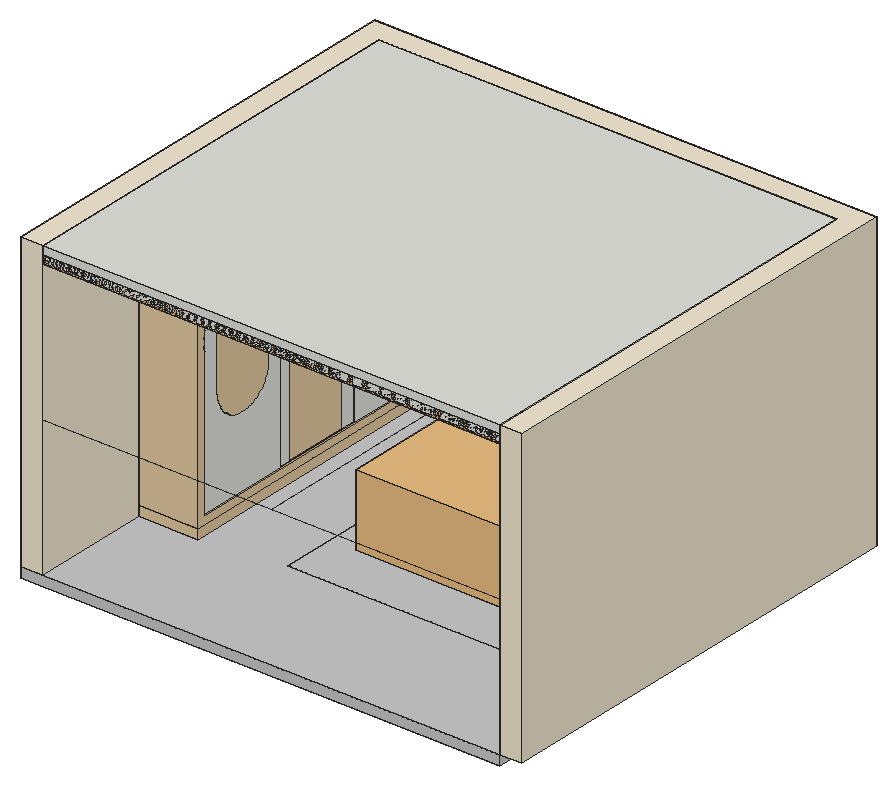
# SketchUp Ruby script. Lengths in inches.
U = 1.inch
M = Sketchup.active_model
def pt(a) = Geom::Point3d.new(a.map { |v| v * U })
def face(e, loops, mat)
  f = e.add_face(loops[0].map { |a| pt(a) })
  loops[1..].each { |l| e.add_face(l.map { |a| pt(a) }).erase! }
  f.material = f.back_material = mat if mat
  f
end
# faces: each face lists its corners as indices into pts; further lists are holes
def faces(e, pts, list, mat = nil) = list.each { |f| face(e, (f[0].is_a?(Array) ? f : [f]).map { |l| l.map { |i| pts[i] } }, mat) }
# xy, xz, yz: faces in a plane at the given z, y or x. An outline is a flat list of corners, or four numbers for a rectangle; further outlines are holes
def ring(l) = l.size == 4 ? [[l[0], l[1]], [l[2], l[1]], [l[2], l[3]], [l[0], l[3]]] : l.each_slice(2).to_a
def flat(e, list, mat, &to3) = list.each { |f| face(e, (f[0].is_a?(Array) ? f : [f]).map { |l| ring(l).map { |u, v| to3.(u, v) } }, mat) }
def xy(e, z, list, mat = nil) = flat(e, list, mat) { |x, y| [x, y, z] }
def xz(e, y, list, mat = nil) = flat(e, list, mat) { |x, z| [x, y, z] }
def yz(e, x, list, mat = nil) = flat(e, list, mat) { |y, z| [x, y, z] }
def lines(e, pts, list) = list.each { |a, b| e.add_line(pt(pts[a]), pt(pts[b])) }
# prism: a flat outline (further loops are holes) pulled along v
def prism(e, loops, v, mat = nil)
  f = face(e, loops, mat); d = Geom::Vector3d.new(v.map { |x| x * U })
  f.pushpull(f.normal.samedirection?(d) ? d.length : -d.length)
end
def box(e, o, s, mat = nil) = prism(e, [[o, [o[0] + s[0], o[1], o[2]], [o[0] + s[0], o[1] + s[1], o[2]], [o[0], o[1] + s[1], o[2]]]], [0, 0, s[2]], mat)
def at(x, y, z, deg = 0) = Geom::Transformation.translation(pt([x, y, z])) * Geom::Transformation.rotation(ORIGIN, Z_AXIS, deg.degrees)
def axes(o, x, y, z) = Geom::Transformation.new([*x, 0, *y, 0, *z, 0, *pt(o).to_a, 1])
def part(name) = M.definitions.add(name)
# library, detail: a bought-in or finely detailed component or shape, given as its bounding box
def library(name, o, s) = part(name).tap { |d| box(d.entities, o, s) }
def detail(e, o, s) = box(e.add_group.entities, o, s)
def put(e, d, t, mat = nil) = e.add_instance(d, t).tap { |i| i.material = mat if mat }
def group(e, t, mat = nil) = e.add_group.tap { |g| g.transformation = t; g.material = mat if mat }.entities
root = M.entities
M.materials.add("0961 AP 7892 PALE IVORY").color = [243, 232, 209]
M.materials.add("0962 AP 9878 Bamboo Straw-N").color = [228, 203, 161]
M.materials.add("Acquerello Marble (TJ07TT)").color = [202, 201, 200]
M.materials.add("Emissive").color = [255, 238, 203]
M.materials.add("Generic").color = [255, 255, 255]
M.materials.add("Kit Kat Speckle_ Stack (OYOLJ5)").color = [227, 224, 217]
M.materials.add("The Belden Brick Company Dapple Gray Matt None Modular (3-5-").color = [200, 200, 200]
M.materials.add("[0130_Gainsboro]").color = [220, 220, 220]
c1 = library("Bed 001",[-37.84,-46.07,0],[75.19,90.39,37.01])
c2 = library("Side Table",[0,-0.77,-1.18],[23.62,18.49,23.93])
c3 = part("Group105\#1")
p = [[0,0,0],[0,0,-46.23],[-14.28,0,-46.23],[93,-56.66,0],[-93,-56.66,0],[93,56.66,0],
  [93,0,0],[-93,56.66,0],[14.28,0,-46.23],[-93,0,0],[0,0,-74.83]]
lines(c3.entities,p,[[0,1],[1,2],[3,4],[5,6],[7,5],[1,8],[9,0],[0,6],[8,10],[4,9],[6,3],[2,10],
  [9,7]])
c4 = part("Rectangle Light\#1")
put(c4.entities,c3,at(0,0,0))
c5 = library("Spot Light",[-5.1,-5.1,-11.05],[10.2,10.2,11.05])
c6 = part("plafonjera+p5")
g1 = group(c6.entities,at(102.27,51.27,12.6))
xy(g1,0,[[[1.84,0,1.6,0.03,1.36,0.09,1.13,0.18,0.91,0.3,0.71,0.45,0.53,0.62,0.375,0.81,0.24,1.02,0.14,1.24,0.0625,1.48,0.02,1.72,0,1.96,0.02,2.21,0.0625,2.45,0.14,2.6875,0.24,2.91,0.375,3.12,0.53,3.3125,0.71,3.48,0.91,3.625,1.13,3.75,1.36,3.84,1.6,3.9,1.84,3.93,2.09,3.93,2.34,3.9,2.58,3.84,2.81,3.75,3.02,3.625,3.22,3.48,3.4,3.3125,3.5625,3.12,3.69,2.91,3.8,2.6875,3.875,2.45,3.92,2.21,3.9375,1.96,3.92,1.72,3.875,1.48,3.8,1.24,3.69,1.02,3.5625,0.81,3.4,0.62,3.22,0.45,3.02,0.3,2.81,0.18,2.58,0.09,2.34,0.03,2.09,0],[1.86,0.2,2.08,0.2,2.3,0.22,2.52,0.28,2.72,0.36,2.92,0.47,3.1,0.6,3.26,0.75,3.4,0.92,3.52,1.11,3.62,1.3125,3.68,1.52,3.73,1.74,3.74,1.96,3.73,2.1875,3.68,2.41,3.62,2.62,3.52,2.82,3.4,3.01,3.26,3.18,3.1,3.33,2.92,3.46,2.72,3.57,2.52,3.65,2.3,3.7,2.08,3.73,1.86,3.73,1.64,3.7,1.42,3.65,1.21,3.57,1.02,3.46,0.84,3.33,0.68,3.18,0.54,3.01,0.42,2.82,0.32,2.62,0.25,2.41,0.21,2.1875,0.2,1.96,0.21,1.74,0.25,1.52,0.32,1.3125,0.42,1.11,0.54,0.92,0.68,0.75,0.84,0.6,1.02,0.47,1.21,0.36,1.42,0.28,1.64,0.22]]],"[0130_Gainsboro]")
xy(g1,0.08,[[1.86,0.2,1.64,0.22,1.42,0.28,1.21,0.36,1.02,0.47,0.84,0.6,0.68,0.75,0.54,0.92,0.42,1.11,0.32,1.3125,0.25,1.52,0.21,1.74,0.2,1.96,0.21,2.1875,0.25,2.41,0.32,2.62,0.42,2.82,0.54,3.01,0.68,3.18,0.84,3.33,1.02,3.46,1.21,3.57,1.42,3.65,1.64,3.7,1.86,3.73,2.08,3.73,2.3,3.7,2.52,3.65,2.72,3.57,2.92,3.46,3.1,3.33,3.26,3.18,3.4,3.01,3.52,2.82,3.62,2.62,3.68,2.41,3.73,2.1875,3.74,1.96,3.73,1.74,3.68,1.52,3.62,1.3125,3.52,1.11,3.4,0.92,3.26,0.75,3.1,0.6,2.92,0.47,2.72,0.36,2.52,0.28,2.3,0.22,2.08,0.2]],"Emissive")
xy(g1,0.39,[[1.84,0,2.09,0,2.34,0.03,2.58,0.09,2.81,0.18,3.02,0.3,3.22,0.45,3.4,0.62,3.5625,0.81,3.69,1.02,3.8,1.24,3.875,1.48,3.92,1.72,3.9375,1.96,3.92,2.21,3.875,2.45,3.8,2.6875,3.69,2.91,3.5625,3.12,3.4,3.3125,3.22,3.48,3.02,3.625,2.81,3.75,2.58,3.84,2.34,3.9,2.09,3.93,1.84,3.93,1.6,3.9,1.36,3.84,1.13,3.75,0.91,3.625,0.71,3.48,0.53,3.3125,0.375,3.12,0.24,2.91,0.14,2.6875,0.0625,2.45,0.02,2.21,0,1.96,0.02,1.72,0.0625,1.48,0.14,1.24,0.24,1.02,0.375,0.81,0.53,0.62,0.71,0.45,0.91,0.3,1.13,0.18,1.36,0.09,1.6,0.03]],"[0130_Gainsboro]")
xz(g1,0,[[1.84,0,2.09,0.39]],"[0130_Gainsboro]")
xz(g1,0.2,[[1.86,0,2.08,0.08]],"[0130_Gainsboro]")
xz(g1,3.73,[[1.86,0,2.08,0.08]],"[0130_Gainsboro]")
xz(g1,3.93,[[1.84,0,2.09,0.39]],"[0130_Gainsboro]")
p = [[1.36,0.09,0],[1.6,0.03,0],[1.6,0.03,0.39],[1.36,0.09,0.39],[1.84,0,0],[1.84,0,0.39],
  [2.09,0,0],[2.34,0.03,0],[2.34,0.03,0.39],[2.09,0,0.39],[2.58,0.09,0],[2.58,0.09,0.39],
  [1.13,0.18,0],[1.13,0.18,0.39],[2.81,0.18,0],[2.81,0.18,0.39],[0.91,0.3,0],[0.91,0.3,0.39],
  [1.64,0.22,0],[1.42,0.28,0],[1.42,0.28,0.08],[1.64,0.22,0.08],[1.86,0.2,0],[1.86,0.2,0.08],
  [2.3,0.22,0],[2.08,0.2,0],[2.08,0.2,0.08],[2.3,0.22,0.08],[2.52,0.28,0],[2.52,0.28,0.08],
  [3.02,0.3,0],[3.02,0.3,0.39],[0.71,0.45,0],[0.71,0.45,0.39],[1.21,0.36,0],[1.21,0.36,0.08],
  [2.72,0.36,0],[2.72,0.36,0.08],[3.22,0.45,0],[3.22,0.45,0.39],[0.53,0.62,0],[0.53,0.62,0.39],
  [1.02,0.47,0],[1.02,0.47,0.08],[2.92,0.47,0],[2.92,0.47,0.08],[3.4,0.62,0],[3.4,0.62,0.39],
  [0.84,0.6,0],[0.84,0.6,0.08],[3.1,0.6,0],[3.1,0.6,0.08],[0.375,0.81,0],[0.375,0.81,0.39],
  [0.68,0.75,0],[0.68,0.75,0.08],[3.26,0.75,0],[3.26,0.75,0.08],[3.5625,0.81,0],[3.5625,0.81,0.39],
  [0.24,1.02,0],[0.24,1.02,0.39],[0.54,0.92,0],[0.54,0.92,0.08],[3.4,0.92,0],[3.4,0.92,0.08],
  [3.69,1.02,0],[3.69,1.02,0.39],[0.42,1.11,0],[0.42,1.11,0.08],[3.52,1.11,0],[3.52,1.11,0.08],
  [0.14,1.24,0],[0.14,1.24,0.39],[3.8,1.24,0],[3.8,1.24,0.39],[0.32,1.3125,0],[0.32,1.3125,0.08],
  [3.62,1.3125,0],[3.62,1.3125,0.08],[0.0625,1.48,0],[0.0625,1.48,0.39],[3.875,1.48,0],[3.875,1.48,0.39],
  [0.25,1.52,0],[0.25,1.52,0.08],[3.68,1.52,0],[3.68,1.52,0.08],[0.02,1.72,0],[0.02,1.72,0.39],
  [0.21,1.74,0],[0.21,1.74,0.08],[3.73,1.74,0],[3.73,1.74,0.08],[3.92,1.72,0],[3.92,1.72,0.39],
  [0,1.96,0],[0,1.96,0.39],[0.2,1.96,0],[0.2,1.96,0.08],[3.74,1.96,0],[3.74,1.96,0.08],
  [3.9375,1.96,0],[3.9375,1.96,0.39],[0.02,2.21,0],[0.02,2.21,0.39],[0.21,2.1875,0],[0.21,2.1875,0.08],
  [3.73,2.1875,0],[3.73,2.1875,0.08],[3.92,2.21,0],[3.92,2.21,0.39],[0.0625,2.45,0],[0.0625,2.45,0.39],
  [0.25,2.41,0],[0.25,2.41,0.08],[3.68,2.41,0],[3.68,2.41,0.08],[3.875,2.45,0],[3.875,2.45,0.39],
  [0.32,2.62,0],[0.32,2.62,0.08],[3.62,2.62,0],[3.62,2.62,0.08],[0.14,2.6875,0],[0.14,2.6875,0.39],
  [3.8,2.6875,0],[3.8,2.6875,0.39],[0.42,2.82,0],[0.42,2.82,0.08],[3.52,2.82,0],[3.52,2.82,0.08],
  [0.24,2.91,0],[0.24,2.91,0.39],[3.69,2.91,0],[3.69,2.91,0.39],[0.54,3.01,0],[0.54,3.01,0.08],
  [3.4,3.01,0],[3.4,3.01,0.08],[0.375,3.12,0],[0.375,3.12,0.39],[3.5625,3.12,0],[3.5625,3.12,0.39],
  [0.68,3.18,0],[0.68,3.18,0.08],[3.26,3.18,0],[3.26,3.18,0.08],[0.53,3.3125,0],[0.53,3.3125,0.39],
  [3.4,3.3125,0],[3.4,3.3125,0.39],[0.84,3.33,0],[0.84,3.33,0.08],[3.1,3.33,0],[3.1,3.33,0.08],
  [0.71,3.48,0],[0.71,3.48,0.39],[1.02,3.46,0],[1.02,3.46,0.08],[2.92,3.46,0],[2.92,3.46,0.08],
  [3.22,3.48,0],[3.22,3.48,0.39],[0.91,3.625,0],[0.91,3.625,0.39],[1.21,3.57,0],[1.21,3.57,0.08],
  [2.72,3.57,0],[2.72,3.57,0.08],[3.02,3.625,0],[3.02,3.625,0.39],[1.13,3.75,0],[1.13,3.75,0.39],
  [1.42,3.65,0],[1.42,3.65,0.08],[1.64,3.7,0],[1.64,3.7,0.08],[2.3,3.7,0],[2.52,3.65,0],
  [2.52,3.65,0.08],[2.3,3.7,0.08],[2.81,3.75,0],[2.81,3.75,0.39],[1.36,3.84,0],[1.36,3.84,0.39],
  [1.86,3.73,0],[1.86,3.73,0.08],[2.08,3.73,0],[2.08,3.73,0.08],[2.58,3.84,0],[2.58,3.84,0.39],
  [1.6,3.9,0],[1.6,3.9,0.39],[2.34,3.9,0],[2.34,3.9,0.39],[1.84,3.93,0],[1.84,3.93,0.39],
  [2.09,3.93,0],[2.09,3.93,0.39]]
faces(g1,p,[[0,1,2,3],[1,4,5,2],[6,7,8,9],[7,10,11,8],[12,0,3,13],[10,14,15,11],[16,12,13,17],[18,19,20,21],
  [22,18,21,23],[24,25,26,27],[28,24,27,29],[14,30,31,15],[32,16,17,33],[19,34,35,20],[36,28,29,37],[30,38,39,31],
  [40,32,33,41],[34,42,43,35],[44,36,37,45],[38,46,47,39],[42,48,49,43],[50,44,45,51],[52,40,41,53],[48,54,55,49],
  [56,50,51,57],[46,58,59,47],[60,52,53,61],[54,62,63,55],[64,56,57,65],[58,66,67,59],[62,68,69,63],[70,64,65,71],
  [72,60,61,73],[66,74,75,67],[68,76,77,69],[78,70,71,79],[80,72,73,81],[74,82,83,75],[76,84,85,77],[86,78,79,87],
  [88,80,81,89],[84,90,91,85],[92,86,87,93],[82,94,95,83],[96,88,89,97],[90,98,99,91],[100,92,93,101],[94,102,103,95],
  [104,96,97,105],[98,106,107,99],[108,100,101,109],[102,110,111,103],[112,104,105,113],[106,114,115,107],[116,108,109,117],[110,118,119,111],
  [114,120,121,115],[122,116,117,123],[124,112,113,125],[118,126,127,119],[120,128,129,121],[130,122,123,131],[132,124,125,133],[126,134,135,127],
  [128,136,137,129],[138,130,131,139],[140,132,133,141],[134,142,143,135],[136,144,145,137],[146,138,139,147],[148,140,141,149],[142,150,151,143],
  [144,152,153,145],[154,146,147,155],[156,148,149,157],[152,158,159,153],[160,154,155,161],[150,162,163,151],[164,156,157,165],[158,166,167,159],
  [168,160,161,169],[162,170,171,163],[172,164,165,173],[166,174,175,167],[174,176,177,175],[178,179,180,181],[179,168,169,180],[170,182,183,171],
  [184,172,173,185],[176,186,187,177],[188,178,181,189],[182,190,191,183],[192,184,185,193],[190,194,195,191],[196,192,193,197],[194,198,199,195]],"[0130_Gainsboro]")
put(g1,c5,at(1.89,2.02,0.07))
c7 = library("ceiling fan",[0,0,0],[76.25,93.13,30.02])
c8 = part("fan")
p = [[217.53,-902.72,540.32],[217.53,-902.72,540.32],[217.53,-902.72,541.35],[217.53,-902.72,541.35]]
lines(c8.entities,p,[[0,1],[2,3]])
put(c8.entities,c7,at(256.45,-350.9,679.41))
c9 = library("Group\#4",[-0.5,-1.92,0],[127,2.42,36])
c10 = library("Group\#18",[-0.5,-0.5,0],[151,1.71,48])
c11 = part("Group8\#1")
xy(c11.entities,7,[[-26.93,80.42,-2.93,81.13],[-26.93,109.26,-2.93,109.97],[-26.93,138.1,-2.93,138.81]])
xy(c11.entities,42.65,[[-26.93,51.9375,-2.93,80.42],[-26.93,81.13,-2.93,109.26],[-26.93,109.97,-2.93,138.1],[-26.93,138.81,-2.93,167.29]])
xy(c11.entities,43.35,[[-26.93,51.9375,-2.93,80.78],[-26.93,80.78,-2.93,109.26],[-26.93,109.97,-2.93,138.45],[-26.93,138.45,-2.93,167.29]])
xy(c11.entities,93,[[-26.93,109.26,-2.93,109.97]])
xz(c11.entities,51.9375,[[-26.93,42.65,-2.93,43.35]])
xz(c11.entities,80.42,[[-26.93,7,-2.93,42.65]])
xz(c11.entities,81.13,[[-26.93,7,-2.93,42.65]])
xz(c11.entities,109.26,[[-26.93,7,-2.93,42.65],[-26.93,43.35,-2.93,93]])
xz(c11.entities,109.97,[[-26.93,7,-2.93,42.65],[-26.93,43.35,-2.93,93]])
xz(c11.entities,138.1,[[-26.93,7,-2.93,42.65]])
xz(c11.entities,138.81,[[-26.93,7,-2.93,42.65]])
xz(c11.entities,167.29,[[-26.93,42.65,-2.93,43.35]])
yz(c11.entities,-26.93,[[80.42,7,80.42,42.65,80.78,43,81.13,42.65,81.13,7],[109.26,7,109.26,42.65,109.61,43,109.97,42.65,109.97,7],[138.1,7,138.1,42.65,138.45,43,138.81,42.65,138.81,7],[51.9375,42.65,51.9375,43.35,80.78,43.35,80.78,43,80.42,42.65],[81.13,42.65,80.78,43,80.78,43.35,109.26,43.35,109.61,43,109.26,42.65],
  [109.97,42.65,109.61,43,109.97,43.35,138.45,43.35,138.45,43,138.1,42.65],[138.81,42.65,138.45,43,138.45,43.35,167.29,43.35,167.29,42.65],[109.61,43,109.26,43.35,109.26,93,109.97,93,109.97,43.35]])
yz(c11.entities,-2.93,[[80.42,7,81.13,7,81.13,42.65,80.78,43,80.42,42.65],[109.26,7,109.97,7,109.97,42.65,109.61,43,109.26,42.65],[138.1,7,138.81,7,138.81,42.65,138.45,43,138.1,42.65],[51.9375,42.65,80.42,42.65,80.78,43,80.78,43.35,51.9375,43.35],[81.13,42.65,109.26,42.65,109.61,43,109.26,43.35,80.78,43.35,80.78,43],
  [109.97,42.65,138.1,42.65,138.45,43,138.45,43.35,109.97,43.35,109.61,43],[138.81,42.65,167.29,42.65,167.29,43.35,138.45,43.35,138.45,43],[109.61,43,109.97,43.35,109.97,93,109.26,93,109.26,43.35]])
c12 = part("Group\#11")
box(c12.entities,[0,0,0],[0.71,37.98,84.58])
c13 = part("Group16\#1")
xy(c13.entities,96,[[-26.22,74.37,-0.64,75.08],[-26.22,98.16,-2.22,98.87],[-26.22,121.95,-2.22,122.65],[-26.22,145.73,-2.22,146.44]])
xy(c13.entities,111.3125,[[-26.22,74.37,-0.64,75.08],[-26.22,98.16,-2.22,98.87],[-26.22,121.95,-2.22,122.65],[-26.22,145.73,-2.22,146.44]])
xz(c13.entities,74.37,[[-26.22,96,-0.64,111.3125]])
xz(c13.entities,75.08,[[-26.22,96,-0.64,111.3125]])
xz(c13.entities,98.16,[[-26.22,96,-2.22,111.3125]])
xz(c13.entities,98.87,[[-26.22,96,-2.22,111.3125]])
xz(c13.entities,121.95,[[-26.22,96,-2.22,111.3125]])
xz(c13.entities,122.65,[[-26.22,96,-2.22,111.3125]])
xz(c13.entities,145.73,[[-26.22,96,-2.22,111.3125]])
xz(c13.entities,146.44,[[-26.22,96,-2.22,111.3125]])
yz(c13.entities,-26.22,[[74.37,96,75.08,111.3125],[98.16,96,98.87,111.3125],[121.95,96,122.65,111.3125],[145.73,96,146.44,111.3125]])
yz(c13.entities,-2.22,[[98.16,96,98.87,111.3125],[121.95,96,122.65,111.3125],[145.73,96,146.44,111.3125]])
yz(c13.entities,-0.64,[[74.37,96,75.08,111.3125]])
c14 = part("Group\#21")
box(c14.entities,[0,0,-0.71],[23.77,15.3125,0.71])
c15 = library("Group\#12",[0,0,-6.6875],[186,171.01,3.47])
c16 = library("Mesh Light\#3",[-0.5,-0.5,-0.1],[1,1,0.2])
xy(root,7,[[12.07,51.9375,34.66,138.45],[34.66,51.9375,36.07,51.9375,36.07,167.29,35.36,167.29,35.36,138.45,34.66,138.45],[12.07,138.45,34.66,167.29],[34.66,138.45,35.36,167.29]])
xy(root,7.71,[[34.66,52.65,35.36,166.58]])
xy(root,7.71,[[35.36,52.65,36.07,166.58]],"0962 AP 9878 Bamboo Straw-N")
xy(root,43,[[12.07,138.45,35.36,167.29]])
xy(root,92.29,[[34.66,52.65,35.36,166.58],[35.36,52.65,36.07,166.58]])
xy(root,93,[[12.07,51.9375,34.66,167.29],[34.66,51.9375,36.07,167.29]])
xy(root,96,[[12.07,48.9375,36.07,170.29]])
xy(root,116.78,[[12,0,198,171]],"0961 AP 7892 PALE IVORY")
xy(root,120,[[12,0,198,171]])
xz(root,0,[[12,113.78,198,116.78],[12,116.78,198,120]])
xz(root,48.9375,[[12.07,4,36.07,96]],"0962 AP 9878 Bamboo Straw-N")
xz(root,51.9375,[[12.07,7,34.66,93],[34.66,7,36.07,93]])
xz(root,52.65,[[34.66,7.71,35.36,92.29],[35.36,7.71,36.07,92.29]])
xz(root,138.45,[[12.07,7,35.36,43]])
xz(root,166.58,[[34.66,7.71,35.36,92.29],[35.36,7.71,36.07,92.29]])
xz(root,167.29,[[12.07,7,34.66,43],[34.66,7,35.36,43],[35.36,7,36.07,7,36.07,93,34.66,93,34.66,43,35.36,43],[12.07,43,34.66,93]])
xz(root,170.29,[[12.07,4,36.07,96]])
xz(root,171,[[12,116.78,198,120]])
yz(root,12,[[0,116.78,171,120]])
yz(root,12.07,[[[48.9375,4,170.29,96],[51.9375,7,167.29,93]],[51.9375,7,80.78,43],[80.78,7,109.61,43],[109.61,7,138.45,43],[51.9375,43,109.61,93],
  [109.61,43,167.29,93]])
yz(root,34.66,[[[51.9375,7,167.29,93],[52.65,7.71,166.58,92.29]]])
yz(root,35.36,[[138.45,7,167.29,7,167.29,43,166.58,43,166.58,7.71,138.45,7.71],[138.45,7.71,166.58,43]])
yz(root,36.07,[[[48.9375,4,170.29,96],[51.9375,7,167.29,93]],[[51.9375,7,167.29,93],[52.65,7.71,166.58,92.29]]],"0962 AP 9878 Bamboo Straw-N")
yz(root,198,[[0,116.78,171,120]])
put(root,c1,axes([119.04,123.37,0.24],[1.04,0,0],[0,1.06,0],[0,0,0.79]))
put(root,c2,axes([166.76,149.48,0],[1.3224,0,0],[0,1.21,0],[0,0,0.6966]))
put(root,c4,axes([105,-0.01,56.66],[1,0,0],[0,0,-1],[0,-1.78143,0]))
put(root,c6,at(-32.13,82.95,103.79))
put(root,c6,at(57.87,82.95,103.79))
put(root,c8,axes([-177.96,384.15,-516.08],[1,0,0],[0,1,0],[0,0,0.89415]))
g2 = group(root,at(36,0,0),"Acquerello Marble (TJ07TT)")
box(g2,[-33,0,-4],[195,171,4])
g3 = group(root,at(27,0,0),"0961 AP 7892 PALE IVORY")
xy(g3,0,[[-24,0,-24,180,180,180,180,0,171,0,171,171,9,171,9,170.29,-15,170.29,-15,0],[9,170.29,45,171]])
xy(g3,36,[[74.51,170.29,135,171]])
xy(g3,120,[[-24,0,-15,0,-15,171,171,171,171,0,180,0,180,180,-24,180]])
xz(g3,0,[[-24,0,-15,120],[171,0,180,120]])
xz(g3,170.29,[[-15,0,45,0,45,11.29,45.81,14.67,47.01,17.94,48.57,21.05,50.49,23.96,52.73,26.62,55.26,29.01,58.06,31.08,61.07,32.82,64.27,34.2,67.61,35.19,71.03,35.8,74.51,36,135,36,135,48.98,134.27,53.67,132.97,58.24,131.12,62.62,128.75,66.73,125.89,70.52,122.58,73.93,118.88,76.91,114.84,79.41,110.53,81.39,106,82.83,101.33,83.71,96.59,84,-15,84]],"Kit Kat Speckle_ Stack (OYOLJ5)")
xz(g3,171,[[9,0,9,84,96.59,84,101.33,83.71,106,82.83,110.53,81.39,114.84,79.41,118.88,76.91,122.58,73.93,125.89,70.52,128.75,66.73,131.12,62.62,132.97,58.24,134.27,53.67,135,48.98,135,36,74.51,36,71.03,35.8,67.61,35.19,64.27,34.2,61.07,32.82,58.06,31.08,55.26,29.01,52.73,26.62,50.49,23.96,48.57,21.05,47.01,17.94,45.81,14.67,45,11.29,45,0],[135,36,171,36,171,120,-15,120,-15,84,96.59,84,101.33,83.71,106,82.83,110.53,81.39,114.84,79.41,118.88,76.91,122.58,73.93,125.89,70.52,128.75,66.73,131.12,62.62,132.97,58.24,134.27,53.67,135,48.98]])
xz(g3,180,[[-24,0,180,120]])
yz(g3,-24,[[0,0,180,120]])
yz(g3,-15,[[0,0,170.29,0,170.29,84,171,84,171,120,0,120]])
yz(g3,45,[[170.29,0,171,11.29]])
yz(g3,171,[[0,0,171,120]])
yz(g3,180,[[0,0,180,120]])
# 1 loose lines left out
p = [[45,171,11.29],[45.81,171,14.67],[45.81,170.29,14.67],[45,170.29,11.29],[47.01,171,17.94],[47.01,170.29,17.94],
  [48.57,171,21.05],[48.57,170.29,21.05],[50.49,171,23.96],[50.49,170.29,23.96],[52.73,171,26.62],[52.73,170.29,26.62],
  [55.26,171,29.01],[55.26,170.29,29.01],[58.06,171,31.08],[58.06,170.29,31.08],[61.07,171,32.82],[61.07,170.29,32.82],
  [64.27,171,34.2],[64.27,170.29,34.2],[67.61,171,35.19],[67.61,170.29,35.19],[71.03,171,35.8],[71.03,170.29,35.8],
  [74.51,171,36],[74.51,170.29,36]]
faces(g3,p,[[0,1,2,3],[1,4,5,2],[4,6,7,5],[6,8,9,7],[8,10,11,9],[10,12,13,11],[12,14,15,13],[14,16,17,15],
  [16,18,19,17],[18,20,21,19],[20,22,23,21],[22,24,25,23]])
put(g3,c9,at(45,171,0))
put(g3,c10,at(-15,170.29,36))
g4 = group(root,at(0,66.51,0))
yz(g4,0,[[0,0,84.09,4]])
g5 = group(root,at(12.07,66.51,4),"0962 AP 9878 Bamboo Straw-N")
box(g5,[0,-17.57,-4],[24,121.35,4])
put(root,c11,at(37.58,0,0))
g6 = group(root,at(35.36,58.65,36.72),"0962 AP 9878 Bamboo Straw-N")
prism(g6,[[[0,8.03,0.99],[0,7.46,1.24],[0,6.73,1.61],[0,6.03,2.02],[0,5.35,2.48],[0,4.71,2.98],[0,4.1,3.52],[0,3.52,4.1],[0,2.98,4.71],[0,2.48,5.35],[0,2.02,6.03],[0,1.61,6.73],[0,1.24,7.46],[0,0.91,8.21],[0,0.64,8.98],[0,0.41,9.76],[0,0.23,10.56],[0,0.1,11.36],[0,0.03,12.17],[0,0,12.99],[0,0,55.57],[0,25.98,55.57],[0,25.98,12.99],[0,25.95,12.17],[0,25.875,11.36],[0,25.75,10.56],[0,25.57,9.76],[0,25.34,8.98],[0,25.07,8.21],[0,24.74,7.46],[0,24.37,6.73],[0,23.96,6.03],[0,23.5,5.35],[0,23,4.71],[0,22.46,4.1],[0,21.88,3.52],[0,21.27,2.98],[0,20.625,2.48],[0,19.95,2.02],[0,19.25,1.61],[0,18.52,1.24],[0,17.95,0.99],[0,17.77,0.91],[0,17,0.64],[0,16.22,0.41],[0,15.42,0.23],[0,14.62,0.1],[0,13.81,0.03],[0,12.99,0],[0,12.17,0.03],[0,11.36,0.1],[0,10.56,0.23],[0,9.76,0.41],[0,8.98,0.64],[0,8.21,0.91]]],[0.75,0,0])
g7 = group(root,at(35.36,52.65,7.71))
box(g7,[0,0,0],[0.71,37.98,84.58])
g8 = group(root,at(34.66,122.6,63.28),"0962 AP 9878 Bamboo Straw-N")
prism(g8,[[[0,-8.03,-0.99],[0,-7.46,-1.24],[0,-6.73,-1.61],[0,-6.03,-2.02],[0,-5.35,-2.48],[0,-4.71,-2.98],[0,-4.1,-3.52],[0,-3.52,-4.1],[0,-2.98,-4.71],[0,-2.48,-5.35],[0,-2.02,-6.03],[0,-1.61,-6.73],[0,-1.24,-7.46],[0,-0.91,-8.21],[0,-0.64,-8.98],[0,-0.41,-9.76],[0,-0.23,-10.56],[0,-0.1,-11.36],[0,-0.03,-12.17],[0,0,-12.99],[0,0,-55.57],[0,-25.98,-55.57],[0,-25.98,-12.99],[0,-25.95,-12.17],[0,-25.875,-11.36],[0,-25.75,-10.56],[0,-25.57,-9.76],[0,-25.34,-8.98],[0,-25.07,-8.21],[0,-24.74,-7.46],[0,-24.37,-6.73],[0,-23.96,-6.03],[0,-23.5,-5.35],[0,-23,-4.71],[0,-22.46,-4.1],[0,-21.88,-3.52],[0,-21.27,-2.98],[0,-20.625,-2.48],[0,-19.95,-2.02],[0,-19.25,-1.61],[0,-18.52,-1.24],[0,-17.95,-0.99],[0,-17.77,-0.91],[0,-17,-0.64],[0,-16.22,-0.41],[0,-15.42,-0.23],[0,-14.62,-0.1],[0,-13.81,-0.03],[0,-12.99,0],[0,-12.17,-0.03],[0,-11.36,-0.1],[0,-10.56,-0.23],[0,-9.76,-0.41],[0,-8.98,-0.64],[0,-8.21,-0.91]]],[0.75,0,0])
put(root,c12,axes([34.66,128.6,92.29],[1,0,0],[0,-1,0],[0,0,-1]))
g9 = group(root,at(35.36,134.6,36.72),"0962 AP 9878 Bamboo Straw-N")
prism(g9,[[[0,8.03,0.99],[0,7.46,1.24],[0,6.73,1.61],[0,6.03,2.02],[0,5.35,2.48],[0,4.71,2.98],[0,4.1,3.52],[0,3.52,4.1],[0,2.98,4.71],[0,2.48,5.35],[0,2.02,6.03],[0,1.61,6.73],[0,1.24,7.46],[0,0.91,8.21],[0,0.64,8.98],[0,0.41,9.76],[0,0.23,10.56],[0,0.1,11.36],[0,0.03,12.17],[0,0,12.99],[0,0,55.57],[0,25.98,55.57],[0,25.98,12.99],[0,25.95,12.17],[0,25.875,11.36],[0,25.75,10.56],[0,25.57,9.76],[0,25.34,8.98],[0,25.07,8.21],[0,24.74,7.46],[0,24.37,6.73],[0,23.96,6.03],[0,23.5,5.35],[0,23,4.71],[0,22.46,4.1],[0,21.88,3.52],[0,21.27,2.98],[0,20.625,2.48],[0,19.95,2.02],[0,19.25,1.61],[0,18.52,1.24],[0,17.95,0.99],[0,17.77,0.91],[0,17,0.64],[0,16.22,0.41],[0,15.42,0.23],[0,14.62,0.1],[0,13.81,0.03],[0,12.99,0],[0,12.17,0.03],[0,11.36,0.1],[0,10.56,0.23],[0,9.76,0.41],[0,8.98,0.64],[0,8.21,0.91]]],[0.75,0,0])
put(root,c12,at(35.36,128.6,7.71))
g10 = group(root,at(12,48.9375,96),"0962 AP 9878 Bamboo Straw-N")
xy(g10,0,[[0.01,0,-0.06,122.0625,24,122.08,24,120.08,0.71,120.0625,0.78,2,24.07,2.01,24.07,0.01]])
xy(g10,15.3125,[[0.78,2,0.71,120.0625,24,120.08,24.07,2.01]])
xy(g10,17.3125,[[0.01,0,24.07,0.01,24,122.08,-0.06,122.0625]])
# 5 loose lines left out
p = [[-0.06,122.0625,0],[0.01,0,0],[0.01,0,17.3125],[-0.06,122.0625,17.3125],[24.07,0.01,0],[24.07,0.01,17.3125],
  [24,120.08,15.3125],[24,120.08,0],[24,122.08,0],[24,122.08,17.3125],[24.07,2.01,0],[24.07,2.01,15.3125],
  [0.78,2,15.3125],[0.78,2,0],[0.71,120.0625,0],[0.71,120.0625,15.3125]]
faces(g10,p,[[0,1,2,3],[1,4,5,2],[6,7,8,9,5,4,10,11],[12,13,14,15],[13,12,11,10],[15,14,7,6],[3,9,8,0]])
put(root,c13,at(36,0,0))
g11 = group(root,at(36.07,50.95,96),"0962 AP 9878 Bamboo Straw-N")
box(g11,[-0.71,0,0],[0.71,23.69,15.3125])
g12 = group(root,at(36.07,74.72,96),"0962 AP 9878 Bamboo Straw-N")
box(g12,[-0.71,0.08,0],[0.71,23.69,15.3125])
put(root,c14,axes([36.07,98.5,96],[0,1,0],[0,0,1],[1,0,0]),"0962 AP 9878 Bamboo Straw-N")
put(root,c14,axes([36.07,122.27,96],[0,1,0],[0,0,1],[1,0,0]),"0962 AP 9878 Bamboo Straw-N")
put(root,c14,axes([36.07,146.05,96],[0,1,0],[0,0,1],[1,0,0]),"0962 AP 9878 Bamboo Straw-N")
put(root,c15,at(12,0,120),"0961 AP 7892 PALE IVORY")
g13 = group(root,at(12,0,120))
xy(g13,0,[[0,0,186,171]])
g14 = group(root,at(63.27,29.25,0),"The Belden Brick Company Dapple Gray Matt None Modular (3-5-")
box(g14,[6,24,0],[91,84,0.24])
g15 = group(root,at(38,170.29,1.5),"Generic")
xz(g15,-0.24,[[14.5,0,15.41,0.03,16.32,0.11,17.22,0.26,18.11,0.46,18.26,0.5,18.98,0.71,19.84,1.02,20.67,1.38,21.49,1.79,22.27,2.26,23.02,2.77,23.74,3.33,24.43,3.93,25.07,4.57,25.67,5.26,26.23,5.98,26.74,6.73,27.21,7.51,27.62,8.33,27.98,9.16,28.29,10.02,28.54,10.89,28.74,11.78,28.89,12.68,28.97,13.59,29,14.5,29,65.5,28.97,66.41,28.89,67.32,28.74,68.22,28.54,69.11,28.29,69.98,27.98,70.84,27.62,71.67,27.21,72.49,26.74,73.27,26.23,74.02,25.67,74.74,25.07,75.43,24.43,76.07,23.74,76.67,23.02,77.23,22.27,77.74,21.49,78.21,20.67,78.62,19.84,78.98,18.98,79.29,18.26,79.5,18.11,79.54,17.22,79.74,16.32,79.89,15.41,79.97,14.5,80,13.59,79.97,12.68,79.89,11.78,79.74,10.89,79.54,10.74,79.5,10.02,79.29,9.16,78.98,8.33,78.62,7.51,78.21,6.73,77.74,5.98,77.23,5.26,76.67,4.57,76.07,3.93,75.43,3.33,74.74,2.77,74.02,2.26,73.27,1.79,72.49,1.38,71.67,1.02,70.84,0.71,69.98,0.46,69.11,0.26,68.22,0.11,67.32,0.03,66.41,0,65.5,0,14.5,0.03,13.59,0.11,12.68,0.26,11.78,0.46,10.89,0.71,10.02,1.02,9.16,1.38,8.33,1.79,7.51,2.26,6.73,2.77,5.98,3.33,5.26,3.93,4.57,4.57,3.93,5.26,3.33,5.98,2.77,6.73,2.26,7.51,1.79,8.33,1.38,9.16,1.02,10.02,0.71,10.74,0.5,10.89,0.46,11.78,0.26,12.68,0.11,13.59,0.03]])
g16 = group(g15,at(0,-0.24,0))
xz(g16,0.24,[[14.5,0,13.59,0.03,12.68,0.11,11.78,0.26,10.89,0.46,10.74,0.5,10.02,0.71,9.16,1.02,8.33,1.38,7.51,1.79,6.73,2.26,5.98,2.77,5.26,3.33,4.57,3.93,3.93,4.57,3.33,5.26,2.77,5.98,2.26,6.73,1.79,7.51,1.38,8.33,1.02,9.16,0.71,10.02,0.46,10.89,0.26,11.78,0.11,12.68,0.03,13.59,0,14.5,0,65.5,0.03,66.41,0.11,67.32,0.26,68.22,0.46,69.11,0.71,69.98,1.02,70.84,1.38,71.67,1.79,72.49,2.26,73.27,2.77,74.02,3.33,74.74,3.93,75.43,4.57,76.07,5.26,76.67,5.98,77.23,6.73,77.74,7.51,78.21,8.33,78.62,9.16,78.98,10.02,79.29,10.74,79.5,10.89,79.54,11.78,79.74,12.68,79.89,13.59,79.97,14.5,80,15.41,79.97,16.32,79.89,17.22,79.74,18.11,79.54,18.26,79.5,18.98,79.29,19.84,78.98,20.67,78.62,21.49,78.21,22.27,77.74,23.02,77.23,23.74,76.67,24.43,76.07,25.07,75.43,25.67,74.74,26.23,74.02,26.74,73.27,27.21,72.49,27.62,71.67,27.98,70.84,28.29,69.98,28.54,69.11,28.74,68.22,28.89,67.32,28.97,66.41,29,65.5,29,14.5,28.97,13.59,28.89,12.68,28.74,11.78,28.54,10.89,28.29,10.02,27.98,9.16,27.62,8.33,27.21,7.51,26.74,6.73,26.23,5.98,25.67,5.26,25.07,4.57,24.43,3.93,23.74,3.33,23.02,2.77,22.27,2.26,21.49,1.79,20.67,1.38,19.84,1.02,18.98,0.71,18.26,0.5,18.11,0.46,17.22,0.26,16.32,0.11,15.41,0.03]])
yz(g16,0,[[0,14.5,0.24,65.5]])
yz(g16,29,[[0,14.5,0.24,65.5]])
p = [[12.68,0.24,0.11],[13.59,0.24,0.03],[13.59,0,0.03],[12.68,0,0.11],[14.5,0.24,0],[14.5,0,0],
  [15.41,0.24,0.03],[15.41,0,0.03],[16.32,0.24,0.11],[16.32,0,0.11],[11.78,0.24,0.26],[11.78,0,0.26],
  [17.22,0.24,0.26],[17.22,0,0.26],[10.89,0.24,0.46],[10.89,0,0.46],[18.11,0.24,0.46],[18.11,0,0.46],
  [10.02,0.24,0.71],[10.74,0.24,0.5],[10.74,0,0.5],[10.02,0,0.71],[18.26,0.24,0.5],[18.26,0,0.5],
  [18.98,0.24,0.71],[18.98,0,0.71],[9.16,0.24,1.02],[9.16,0,1.02],[19.84,0.24,1.02],[19.84,0,1.02],
  [8.33,0.24,1.38],[8.33,0,1.38],[20.67,0.24,1.38],[20.67,0,1.38],[7.51,0.24,1.79],[7.51,0,1.79],
  [21.49,0.24,1.79],[21.49,0,1.79],[6.73,0.24,2.26],[6.73,0,2.26],[22.27,0.24,2.26],[22.27,0,2.26],
  [5.98,0.24,2.77],[5.98,0,2.77],[23.02,0.24,2.77],[23.02,0,2.77],[5.26,0.24,3.33],[5.26,0,3.33],
  [23.74,0.24,3.33],[23.74,0,3.33],[4.57,0.24,3.93],[4.57,0,3.93],[24.43,0.24,3.93],[24.43,0,3.93],
  [3.93,0.24,4.57],[3.93,0,4.57],[25.07,0.24,4.57],[25.07,0,4.57],[3.33,0.24,5.26],[3.33,0,5.26],
  [25.67,0.24,5.26],[25.67,0,5.26],[2.77,0.24,5.98],[2.77,0,5.98],[26.23,0.24,5.98],[26.23,0,5.98],
  [2.26,0.24,6.73],[2.26,0,6.73],[26.74,0.24,6.73],[26.74,0,6.73],[1.79,0.24,7.51],[1.79,0,7.51],
  [27.21,0.24,7.51],[27.21,0,7.51],[1.38,0.24,8.33],[1.38,0,8.33],[27.62,0.24,8.33],[27.62,0,8.33],
  [1.02,0.24,9.16],[1.02,0,9.16],[27.98,0.24,9.16],[27.98,0,9.16],[0.71,0.24,10.02],[0.71,0,10.02],
  [28.29,0.24,10.02],[28.29,0,10.02],[0.46,0.24,10.89],[0.46,0,10.89],[28.54,0.24,10.89],[28.54,0,10.89],
  [0.26,0.24,11.78],[0.26,0,11.78],[28.74,0.24,11.78],[28.74,0,11.78],[0.11,0.24,12.68],[0.11,0,12.68],
  [28.89,0.24,12.68],[28.89,0,12.68],[0.03,0.24,13.59],[0.03,0,13.59],[28.97,0.24,13.59],[28.97,0,13.59],
  [0,0.24,14.5],[0,0,14.5],[29,0.24,14.5],[29,0,14.5],[0.03,0.24,66.41],[0,0.24,65.5],
  [0,0,65.5],[0.03,0,66.41],[29,0.24,65.5],[28.97,0.24,66.41],[28.97,0,66.41],[29,0,65.5],
  [0.11,0.24,67.32],[0.11,0,67.32],[28.89,0.24,67.32],[28.89,0,67.32],[0.26,0.24,68.22],[0.26,0,68.22],
  [28.74,0.24,68.22],[28.74,0,68.22],[0.46,0.24,69.11],[0.46,0,69.11],[28.54,0.24,69.11],[28.54,0,69.11],
  [0.71,0.24,69.98],[0.71,0,69.98],[28.29,0.24,69.98],[28.29,0,69.98],[1.02,0.24,70.84],[1.02,0,70.84],
  [27.98,0.24,70.84],[27.98,0,70.84],[1.38,0.24,71.67],[1.38,0,71.67],[27.62,0.24,71.67],[27.62,0,71.67],
  [1.79,0.24,72.49],[1.79,0,72.49],[27.21,0.24,72.49],[27.21,0,72.49],[2.26,0.24,73.27],[2.26,0,73.27],
  [26.74,0.24,73.27],[26.74,0,73.27],[2.77,0.24,74.02],[2.77,0,74.02],[26.23,0.24,74.02],[26.23,0,74.02],
  [3.33,0.24,74.74],[3.33,0,74.74],[25.67,0.24,74.74],[25.67,0,74.74],[3.93,0.24,75.43],[3.93,0,75.43],
  [25.07,0.24,75.43],[25.07,0,75.43],[4.57,0.24,76.07],[4.57,0,76.07],[24.43,0.24,76.07],[24.43,0,76.07],
  [5.26,0.24,76.67],[5.26,0,76.67],[23.74,0.24,76.67],[23.74,0,76.67],[5.98,0.24,77.23],[5.98,0,77.23],
  [23.02,0.24,77.23],[23.02,0,77.23],[6.73,0.24,77.74],[6.73,0,77.74],[22.27,0.24,77.74],[22.27,0,77.74],
  [7.51,0.24,78.21],[7.51,0,78.21],[21.49,0.24,78.21],[21.49,0,78.21],[8.33,0.24,78.62],[8.33,0,78.62],
  [20.67,0.24,78.62],[20.67,0,78.62],[9.16,0.24,78.98],[9.16,0,78.98],[19.84,0.24,78.98],[19.84,0,78.98],
  [10.02,0.24,79.29],[10.02,0,79.29],[18.98,0.24,79.29],[18.98,0,79.29],[10.74,0.24,79.5],[10.74,0,79.5],
  [18.26,0.24,79.5],[18.26,0,79.5],[10.89,0.24,79.54],[10.89,0,79.54],[11.78,0.24,79.74],[11.78,0,79.74],
  [18.11,0.24,79.54],[17.22,0.24,79.74],[17.22,0,79.74],[18.11,0,79.54],[12.68,0.24,79.89],[12.68,0,79.89],
  [16.32,0.24,79.89],[16.32,0,79.89],[13.59,0.24,79.97],[13.59,0,79.97],[15.41,0.24,79.97],[15.41,0,79.97],
  [14.5,0.24,80],[14.5,0,80]]
faces(g16,p,[[0,1,2,3],[1,4,5,2],[4,6,7,5],[6,8,9,7],[10,0,3,11],[8,12,13,9],[14,10,11,15],[12,16,17,13],
  [18,19,20,21],[19,14,15,20],[16,22,23,17],[22,24,25,23],[26,18,21,27],[24,28,29,25],[30,26,27,31],[28,32,33,29],
  [34,30,31,35],[32,36,37,33],[38,34,35,39],[36,40,41,37],[42,38,39,43],[40,44,45,41],[46,42,43,47],[44,48,49,45],
  [50,46,47,51],[48,52,53,49],[54,50,51,55],[52,56,57,53],[58,54,55,59],[56,60,61,57],[62,58,59,63],[60,64,65,61],
  [66,62,63,67],[64,68,69,65],[70,66,67,71],[68,72,73,69],[74,70,71,75],[72,76,77,73],[78,74,75,79],[76,80,81,77],
  [82,78,79,83],[80,84,85,81],[86,82,83,87],[84,88,89,85],[90,86,87,91],[88,92,93,89],[94,90,91,95],[92,96,97,93],
  [98,94,95,99],[96,100,101,97],[102,98,99,103],[100,104,105,101],[106,107,108,109],[110,111,112,113],[114,106,109,115],[111,116,117,112],
  [118,114,115,119],[116,120,121,117],[122,118,119,123],[120,124,125,121],[126,122,123,127],[124,128,129,125],[130,126,127,131],[128,132,133,129],
  [134,130,131,135],[132,136,137,133],[138,134,135,139],[136,140,141,137],[142,138,139,143],[140,144,145,141],[146,142,143,147],[144,148,149,145],
  [150,146,147,151],[148,152,153,149],[154,150,151,155],[152,156,157,153],[158,154,155,159],[156,160,161,157],[162,158,159,163],[160,164,165,161],
  [166,162,163,167],[164,168,169,165],[170,166,167,171],[168,172,173,169],[174,170,171,175],[172,176,177,173],[178,174,175,179],[176,180,181,177],
  [182,178,179,183],[180,184,185,181],[186,182,183,187],[184,188,189,185],[190,186,187,191],[188,192,193,189],[194,190,191,195],[196,194,195,197],
  [198,199,200,201],[192,198,201,193],[202,196,197,203],[199,204,205,200],[206,202,203,207],[204,208,209,205],[210,206,207,211],[208,210,211,209]])
put(g16,c16,axes([14.5,0.12,40],[30,0,0],[0,1.23622,0],[0,0,81]))
